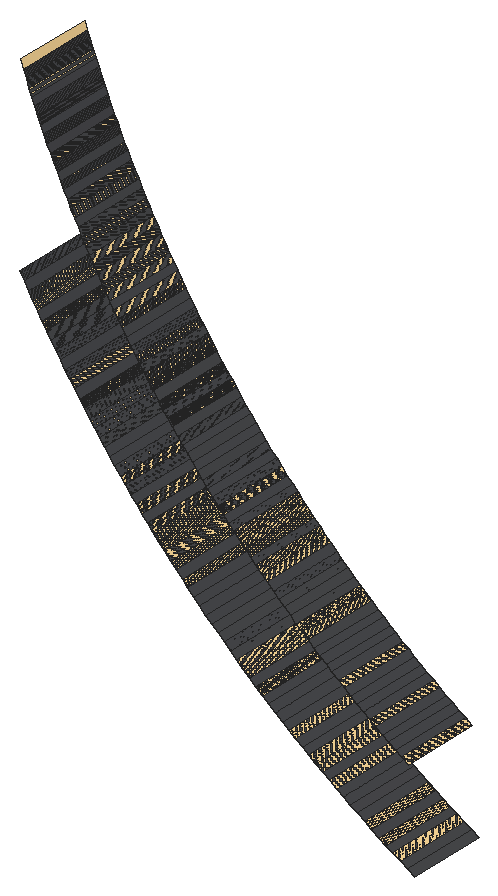
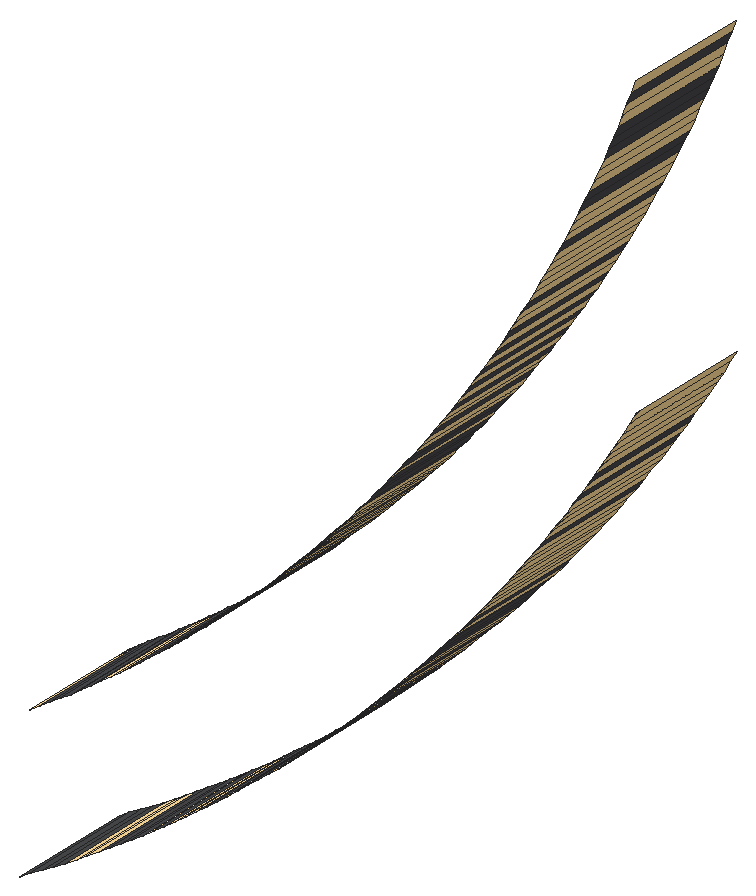
# SketchUp Ruby script. Lengths in inches.
U = 1.inch
M = Sketchup.active_model
def pt(a) = Geom::Point3d.new(a.map { |v| v * U })
def face(e, loops, mat)
  f = e.add_face(loops[0].map { |a| pt(a) })
  loops[1..].each { |l| e.add_face(l.map { |a| pt(a) }).erase! }
  f.material = f.back_material = mat if mat
  f
end
# faces: each face lists its corners as indices into pts; further lists are holes
def faces(e, pts, list, mat = nil) = list.each { |f| face(e, (f[0].is_a?(Array) ? f : [f]).map { |l| l.map { |i| pts[i] } }, mat) }
# xy, xz, yz: faces in a plane at the given z, y or x. An outline is a flat list of corners, or four numbers for a rectangle; further outlines are holes
def ring(l) = l.size == 4 ? [[l[0], l[1]], [l[2], l[1]], [l[2], l[3]], [l[0], l[3]]] : l.each_slice(2).to_a
def flat(e, list, mat, &to3) = list.each { |f| face(e, (f[0].is_a?(Array) ? f : [f]).map { |l| ring(l).map { |u, v| to3.(u, v) } }, mat) }
def xy(e, z, list, mat = nil) = flat(e, list, mat) { |x, y| [x, y, z] }
def xz(e, y, list, mat = nil) = flat(e, list, mat) { |x, z| [x, y, z] }
def yz(e, x, list, mat = nil) = flat(e, list, mat) { |y, z| [x, y, z] }
def lines(e, pts, list) = list.each { |a, b| e.add_line(pt(pts[a]), pt(pts[b])) }
# prism: a flat outline (further loops are holes) pulled along v
def prism(e, loops, v, mat = nil)
  f = face(e, loops, mat); d = Geom::Vector3d.new(v.map { |x| x * U })
  f.pushpull(f.normal.samedirection?(d) ? d.length : -d.length)
end
def box(e, o, s, mat = nil) = prism(e, [[o, [o[0] + s[0], o[1], o[2]], [o[0] + s[0], o[1] + s[1], o[2]], [o[0], o[1] + s[1], o[2]]]], [0, 0, s[2]], mat)
def at(x, y, z, deg = 0) = Geom::Transformation.translation(pt([x, y, z])) * Geom::Transformation.rotation(ORIGIN, Z_AXIS, deg.degrees)
def axes(o, x, y, z) = Geom::Transformation.new([*x, 0, *y, 0, *z, 0, *pt(o).to_a, 1])
def part(name) = M.definitions.add(name)
# library, detail: a bought-in or finely detailed component or shape, given as its bounding box
def library(name, o, s) = part(name).tap { |d| box(d.entities, o, s) }
def detail(e, o, s) = box(e.add_group.entities, o, s)
def put(e, d, t, mat = nil) = e.add_instance(d, t).tap { |i| i.material = mat if mat }
def group(e, t, mat = nil) = e.add_group.tap { |g| g.transformation = t; g.material = mat if mat }.entities
root = M.entities
M.materials.add("1432 AP 8245 TAR ROAD").color = [71, 72, 75]
M.materials.add("Outer Light").color = [251, 217, 152]
p = [[268.43,95.37,447.23],[268.56,95.37,447.15],[268.56,96.87,447.15],[268.43,96.87,447.23],[268.29,95.37,447.3125],[268.29,96.87,447.3125],
  [268.29,96.87,447.3125],[268.43,96.87,447.23],[268.43,95.37,447.23],[268.29,95.37,447.3125],[268.15,95.37,447.4],[268.15,96.87,447.4],
  [268.15,96.87,447.4],[268.15,95.37,447.4],[268.02,95.37,447.48],[268.02,96.87,447.48],[268.02,96.87,447.48],[268.02,95.37,447.48],
  [267.88,95.37,447.57],[267.88,96.87,447.57],[267.88,96.87,447.57],[267.88,95.37,447.57],[267.75,95.37,447.66],[267.75,96.87,447.66],
  [267.75,96.87,447.66],[267.75,95.37,447.66],[267.48,95.37,447.84],[267.61,95.37,447.75],[267.61,96.87,447.75],[267.48,96.87,447.84],
  [267.48,96.87,447.84],[267.61,96.87,447.75],[267.61,95.37,447.75],[267.48,95.37,447.84],[267.34,95.37,447.93],[267.34,96.87,447.93],
  [267.34,96.87,447.93],[267.34,95.37,447.93],[267.21,95.37,448.02],[267.21,96.87,448.02],[267.21,96.87,448.02],[267.21,95.37,448.02],
  [267.08,95.37,448.11],[267.08,96.87,448.11],[267.08,96.87,448.11],[267.08,95.37,448.11],[266.95,95.37,448.21],[266.95,96.87,448.21],
  [266.95,96.87,448.21],[266.95,95.37,448.21],[266.82,95.37,448.3],[266.82,96.87,448.3],[266.82,96.87,448.3],[266.82,95.37,448.3],
  [266.69,95.37,448.4],[266.69,96.87,448.4],[266.69,96.87,448.4],[266.69,95.37,448.4],[266.5625,95.37,448.5],[266.5625,96.87,448.5],
  [266.5625,96.87,448.5],[266.5625,95.37,448.5],[266.44,95.37,448.59],[266.44,96.87,448.59],[266.44,96.87,448.59],[266.44,95.37,448.59],
  [266.31,95.37,448.69],[266.31,96.87,448.69],[266.31,96.87,448.69],[266.31,95.37,448.69],[266.18,95.37,448.79],[266.18,96.87,448.79],
  [266.18,96.87,448.79],[266.18,95.37,448.79],[266.06,95.37,448.89],[266.06,96.87,448.89],[266.06,96.87,448.89],[266.06,95.37,448.89],
  [265.93,95.37,449],[265.93,96.87,449],[265.93,96.87,449],[265.93,95.37,449],[265.81,95.37,449.1],[265.81,96.87,449.1],
  [265.81,96.87,449.1],[265.81,95.37,449.1],[268.44,96.87,448.99],[268.32,96.87,449.08],[268.32,95.37,449.08],[268.44,95.37,448.99],
  [268.44,95.37,448.99],[268.32,95.37,449.08],[268.32,96.87,449.08],[268.44,96.87,448.99],[265.6875,95.37,449.2],[265.6875,96.87,449.2],
  [265.6875,96.87,449.2],[265.6875,95.37,449.2],[268.2,96.87,449.16],[268.2,95.37,449.16],[268.2,95.37,449.16],[268.2,96.87,449.16],
  [265.5625,95.37,449.31],[265.5625,96.87,449.31],[265.5625,96.87,449.31],[265.5625,95.37,449.31],[268.07,96.87,449.25],[267.95,96.87,449.33],
  [267.95,95.37,449.33],[268.07,95.37,449.25],[268.07,95.37,449.25],[267.95,95.37,449.33],[267.95,96.87,449.33],[268.07,96.87,449.25],
  [265.44,95.37,449.41],[265.44,96.87,449.41],[265.44,96.87,449.41],[265.44,95.37,449.41],[267.83,96.87,449.42],[267.83,95.37,449.42],
  [267.83,95.37,449.42],[267.83,96.87,449.42],[265.32,95.37,449.52],[265.32,96.87,449.52],[265.32,96.87,449.52],[265.32,95.37,449.52],
  [267.71,96.87,449.51],[267.71,95.37,449.51],[267.71,95.37,449.51],[267.71,96.87,449.51],[265.2,95.37,449.63],[265.2,96.87,449.63],
  [265.2,96.87,449.63],[265.2,95.37,449.63],[267.59,96.87,449.6],[267.59,95.37,449.6],[267.59,95.37,449.6],[267.59,96.87,449.6],
  [265.08,95.37,449.74],[265.08,96.87,449.74],[265.08,96.87,449.74],[265.08,95.37,449.74],[267.47,96.87,449.6875],[267.47,95.37,449.6875],
  [267.47,95.37,449.6875],[267.47,96.87,449.6875],[264.97,95.37,449.85],[264.97,96.87,449.85],[264.97,96.87,449.85],[264.97,95.37,449.85],
  [267.35,96.87,449.78],[267.35,95.37,449.78],[267.35,95.37,449.78],[267.35,96.87,449.78],[264.85,95.37,449.96],[264.85,96.87,449.96],
  [264.85,96.87,449.96],[264.85,95.37,449.96],[267.24,96.87,449.87],[267.24,95.37,449.87],[267.24,95.37,449.87],[267.24,96.87,449.87],
  [267.12,96.87,449.96],[267.12,95.37,449.96],[267.12,95.37,449.96],[267.12,96.87,449.96],[264.73,95.37,450.07],[264.73,96.87,450.07],
  [264.73,96.87,450.07],[264.73,95.37,450.07],[267,96.87,450.06],[267,95.37,450.06],[267,95.37,450.06],[267,96.87,450.06],
  [264.62,95.37,450.18],[264.62,96.87,450.18],[264.62,96.87,450.18],[264.62,95.37,450.18],[266.89,96.87,450.15],[266.89,95.37,450.15],
  [266.89,95.37,450.15],[266.89,96.87,450.15],[264.5,95.37,450.3],[264.5,96.87,450.3],[264.5,96.87,450.3],[264.5,95.37,450.3],
  [266.77,96.87,450.25],[266.66,96.87,450.34],[266.66,95.37,450.34],[266.77,95.37,450.25],[266.77,95.37,450.25],[266.66,95.37,450.34],
  [266.66,96.87,450.34],[266.77,96.87,450.25],[264.39,95.37,450.41],[264.39,96.87,450.41],[264.39,96.87,450.41],[264.39,95.37,450.41],
  [266.55,96.87,450.44],[266.55,95.37,450.44],[266.55,95.37,450.44],[266.55,96.87,450.44],[264.28,95.37,450.53],[264.28,96.87,450.53],
  [264.28,96.87,450.53],[264.28,95.37,450.53],[266.44,96.87,450.54],[266.44,95.37,450.54],[266.44,95.37,450.54],[266.44,96.87,450.54],
  [264.17,95.37,450.64],[264.17,96.87,450.64],[264.17,96.87,450.64],[264.17,95.37,450.64],[266.32,96.87,450.64],[266.32,95.37,450.64],
  [266.32,95.37,450.64],[266.32,96.87,450.64],[264.06,95.37,450.76],[264.06,96.87,450.76],[264.06,96.87,450.76],[264.06,95.37,450.76],
  [266.21,96.87,450.74],[266.21,95.37,450.74],[266.21,95.37,450.74],[266.21,96.87,450.74],[266.1,96.87,450.84],[266.1,95.37,450.84],
  [266.1,95.37,450.84],[266.1,96.87,450.84],[263.95,95.37,450.875],[263.95,96.87,450.875],[263.95,96.87,450.875],[263.95,95.37,450.875],
  [265.99,96.87,450.94],[265.99,95.37,450.94],[265.99,95.37,450.94],[265.99,96.87,450.94],[263.84,95.37,451],[263.84,96.87,451],
  [263.84,96.87,451],[263.84,95.37,451],[265.89,96.87,451.04],[265.89,95.37,451.04],[265.89,95.37,451.04],[265.89,96.87,451.04],
  [263.73,95.37,451.11],[263.73,96.87,451.11],[263.73,96.87,451.11],[263.73,95.37,451.11],[265.78,96.87,451.15],[265.78,95.37,451.15],
  [265.78,95.37,451.15],[265.78,96.87,451.15],[263.62,95.37,451.24],[263.62,96.87,451.24],[263.62,96.87,451.24],[263.62,95.37,451.24],
  [265.67,96.87,451.25],[265.67,95.37,451.25],[265.67,95.37,451.25],[265.67,96.87,451.25],[263.52,95.37,451.36],[263.52,96.87,451.36],
  [263.52,96.87,451.36],[263.52,95.37,451.36],[265.56,96.87,451.36],[265.56,95.37,451.36],[265.56,95.37,451.36],[265.56,96.87,451.36],
  [263.41,95.37,451.48],[263.41,96.87,451.48],[263.41,96.87,451.48],[263.41,95.37,451.48],[265.46,96.87,451.46],[265.46,95.37,451.46],
  [265.46,95.37,451.46],[265.46,96.87,451.46],[263.31,95.37,451.6],[263.31,96.87,451.6],[263.31,96.87,451.6],[263.31,95.37,451.6],
  [265.36,96.87,451.57],[265.36,95.37,451.57],[265.36,95.37,451.57],[265.36,96.87,451.57],[263.2,95.37,451.72],[263.2,96.87,451.72],
  [263.2,96.87,451.72],[263.2,95.37,451.72],[265.25,96.87,451.68],[265.25,95.37,451.68],[265.25,95.37,451.68],[265.25,96.87,451.68],
  [263.1,95.37,451.85],[263.1,96.87,451.85],[263.1,96.87,451.85],[263.1,95.37,451.85],[265.15,96.87,451.79],[265.15,95.37,451.79],
  [265.15,95.37,451.79],[265.15,96.87,451.79],[263,95.37,451.97],[263,96.87,451.97],[263,96.87,451.97],[263,95.37,451.97],
  [265.05,96.87,451.89],[265.05,95.37,451.89],[265.05,95.37,451.89],[265.05,96.87,451.89],[264.95,96.87,452],[264.95,95.37,452],
  [264.95,95.37,452],[264.95,96.87,452],[262.9,95.37,452.1],[262.9,96.87,452.1],[262.9,96.87,452.1],[262.9,95.37,452.1],
  [264.85,96.87,452.12],[264.85,95.37,452.12],[264.85,95.37,452.12],[264.85,96.87,452.12],[262.8,95.37,452.23],[262.8,96.87,452.23],
  [262.8,96.87,452.23],[262.8,95.37,452.23],[264.75,96.87,452.23],[264.75,95.37,452.23],[264.75,95.37,452.23],[264.75,96.87,452.23],
  [262.7,95.37,452.36],[262.7,96.87,452.36],[262.7,96.87,452.36],[262.7,95.37,452.36],[264.65,96.87,452.34],[264.65,95.37,452.34],
  [264.65,95.37,452.34],[264.65,96.87,452.34],[264.55,96.87,452.45],[264.55,95.37,452.45],[264.55,95.37,452.45],[264.55,96.87,452.45],
  [262.61,95.37,452.48],[262.61,96.87,452.48],[262.61,96.87,452.48],[262.61,95.37,452.48],[262.51,95.37,452.61],[262.51,96.87,452.61],
  [262.51,96.87,452.61],[262.51,95.37,452.61],[264.46,96.87,452.57],[264.46,95.37,452.57],[264.46,95.37,452.57],[264.46,96.87,452.57],
  [262.42,95.37,452.74],[262.42,96.87,452.74],[262.42,96.87,452.74],[262.42,95.37,452.74],[264.36,96.87,452.68],[264.36,95.37,452.68],
  [264.36,95.37,452.68],[264.36,96.87,452.68],[262.32,95.37,452.875],[262.32,96.87,452.875],[262.32,96.87,452.875],[262.32,95.37,452.875],
  [264.27,96.87,452.8],[264.27,95.37,452.8],[264.27,95.37,452.8],[264.27,96.87,452.8],[264.17,96.87,452.91],[264.17,95.37,452.91],
  [264.17,95.37,452.91],[264.17,96.87,452.91],[262.23,95.37,453],[262.23,96.87,453],[262.23,96.87,453],[262.23,95.37,453],
  [264.08,96.87,453.03],[264.08,95.37,453.03],[264.08,95.37,453.03],[264.08,96.87,453.03],[262.14,95.37,453.14],[262.14,96.87,453.14],
  [262.14,96.87,453.14],[262.14,95.37,453.14],[263.99,96.87,453.15],[263.99,95.37,453.15],[263.99,95.37,453.15],[263.99,96.87,453.15],
  [262.04,95.37,453.27],[262.04,96.87,453.27],[262.04,96.87,453.27],[262.04,95.37,453.27],[263.9,96.87,453.27],[263.9,95.37,453.27],
  [263.9,95.37,453.27],[263.9,96.87,453.27],[261.95,95.37,453.4],[261.95,96.87,453.4],[261.95,96.87,453.4],[261.95,95.37,453.4],
  [263.81,96.87,453.38],[263.81,95.37,453.38],[263.81,95.37,453.38],[263.81,96.87,453.38],[261.87,95.37,453.54],[261.87,96.87,453.54],
  [261.87,96.87,453.54],[261.87,95.37,453.54],[263.72,96.87,453.5],[263.72,95.37,453.5],[263.72,95.37,453.5],[263.72,96.87,453.5],
  [261.78,95.37,453.67],[261.78,96.87,453.67],[261.78,96.87,453.67],[261.78,95.37,453.67],[263.63,96.87,453.625],[263.63,95.37,453.625],
  [263.63,95.37,453.625],[263.63,96.87,453.625],[263.54,96.87,453.75],[263.54,95.37,453.75],[263.54,95.37,453.75],[263.54,96.87,453.75],
  [261.69,95.37,453.81],[261.69,96.87,453.81],[261.69,96.87,453.81],[261.69,95.37,453.81],[263.46,96.87,453.87],[263.46,95.37,453.87],
  [263.46,95.37,453.87],[263.46,96.87,453.87],[261.61,95.37,453.94],[261.61,96.87,453.94],[261.61,96.87,453.94],[261.61,95.37,453.94],
  [261.52,95.37,454.08],[261.52,96.87,454.08],[261.52,96.87,454.08],[261.52,95.37,454.08],[263.37,96.87,453.99],[263.37,95.37,453.99],
  [263.37,95.37,453.99],[263.37,96.87,453.99],[263.29,96.87,454.11],[263.29,95.37,454.11],[263.29,95.37,454.11],[263.29,96.87,454.11],
  [261.4375,95.37,454.22],[261.4375,96.87,454.22],[261.4375,96.87,454.22],[261.4375,95.37,454.22],[263.2,96.87,454.24],[263.2,95.37,454.24],
  [263.2,95.37,454.24],[263.2,96.87,454.24],[261.35,95.37,454.36],[261.35,96.87,454.36],[261.35,96.87,454.36],[261.35,95.37,454.36],
  [263.12,96.87,454.36],[263.12,95.37,454.36],[263.12,95.37,454.36],[263.12,96.87,454.36],[261.27,95.37,454.5],[261.27,96.87,454.5],
  [261.27,96.87,454.5],[261.27,95.37,454.5],[263.04,96.87,454.49],[263.04,95.37,454.49],[263.04,95.37,454.49],[263.04,96.87,454.49],
  [261.19,95.37,454.64],[261.19,96.87,454.64],[261.19,96.87,454.64],[261.19,95.37,454.64],[262.96,96.87,454.61],[262.96,95.37,454.61],
  [262.96,95.37,454.61],[262.96,96.87,454.61],[261.11,95.37,454.78],[261.11,96.87,454.78],[261.11,96.87,454.78],[261.11,95.37,454.78],
  [262.88,96.87,454.74],[262.88,95.37,454.74],[262.88,95.37,454.74],[262.88,96.87,454.74],[262.8,96.87,454.86],[262.8,95.37,454.86],
  [262.8,95.37,454.86],[262.8,96.87,454.86],[262.72,96.87,454.99],[262.72,95.37,454.99],[262.72,95.37,454.99],[262.72,96.87,454.99],
  [262.65,96.87,455.12],[262.65,95.37,455.12],[262.65,95.37,455.12],[262.65,96.87,455.12],[262.57,96.87,455.25],[262.57,95.37,455.25],
  [262.57,95.37,455.25],[262.57,96.87,455.25],[262.5,96.87,455.38],[262.5,95.37,455.38],[262.5,95.37,455.38],[262.5,96.87,455.38],
  [262.42,96.87,455.51],[262.42,95.37,455.51],[262.42,95.37,455.51],[262.42,96.87,455.51],[262.35,96.87,455.64],[262.35,95.37,455.64],
  [262.35,95.37,455.64],[262.35,96.87,455.64],[262.28,96.87,455.77],[262.28,95.37,455.77],[262.28,95.37,455.77],[262.28,96.87,455.77],
  [262.21,96.87,455.9],[262.21,95.37,455.9],[262.21,95.37,455.9],[262.21,96.87,455.9],[262.14,96.87,456.03],[262.14,95.37,456.03],
  [262.14,95.37,456.03],[262.14,96.87,456.03],[262.07,96.87,456.17],[262.07,95.37,456.17],[262.07,95.37,456.17],[262.07,96.87,456.17],
  [262,96.87,456.3],[262,95.37,456.3],[262,95.37,456.3],[262,96.87,456.3],[261.9375,96.87,456.43],[261.9375,95.37,456.43],
  [261.9375,95.37,456.43],[261.9375,96.87,456.43],[261.87,96.87,456.57],[261.87,95.37,456.57],[261.87,95.37,456.57],[261.87,96.87,456.57],
  [261.81,96.87,456.7],[261.81,95.37,456.7],[261.81,95.37,456.7],[261.81,96.87,456.7],[261.75,96.87,456.84],[261.75,95.37,456.84],
  [261.75,95.37,456.84],[261.75,96.87,456.84],[261.68,96.87,456.97],[261.68,95.37,456.97],[261.68,95.37,456.97],[261.68,96.87,456.97],
  [261.62,96.87,457.11],[261.62,95.37,457.11],[261.62,95.37,457.11],[261.62,96.87,457.11],[261.5625,96.87,457.25],[261.5625,95.37,457.25],
  [261.5625,95.37,457.25],[261.5625,96.87,457.25],[261.5,96.87,457.38],[261.5,95.37,457.38],[261.5,95.37,457.38],[261.5,96.87,457.38],
  [261.45,96.87,457.52],[261.45,95.37,457.52],[261.45,95.37,457.52],[261.45,96.87,457.52],[261.39,96.87,457.66],[261.39,95.37,457.66],
  [261.39,95.37,457.66],[261.39,96.87,457.66],[261.33,96.87,457.8],[261.33,95.37,457.8],[261.33,95.37,457.8],[261.33,96.87,457.8],
  [261.28,96.87,457.9375],[261.28,95.37,457.9375],[261.28,95.37,457.9375],[261.28,96.87,457.9375],[261.23,96.87,458.08],[261.23,95.37,458.08],
  [261.23,95.37,458.08],[261.23,96.87,458.08],[261.17,96.87,458.22],[261.17,95.37,458.22],[261.17,95.37,458.22],[261.17,96.87,458.22],
  [261.125,96.87,458.36],[261.125,95.37,458.36]]
faces(root,p,[[0,1,2,3],[4,0,3,5],[10,4,5,11],[14,10,11,15],[18,14,15,19],[22,18,19,23],[26,27,28,29],[27,22,23,28],
  [34,26,29,35],[38,34,35,39],[42,38,39,43],[46,42,43,47],[50,46,47,51],[54,50,51,55],[58,54,55,59],[62,58,59,63],
  [66,62,63,67],[70,66,67,71],[74,70,71,75],[78,74,75,79],[82,78,79,83],[90,91,92,93],[94,82,83,95],[91,100,101,92],
  [102,94,95,103],[110,111,112,113],[100,110,113,101],[114,102,103,115],[111,120,121,112],[122,114,115,123],[120,128,129,121],[130,122,123,131],
  [128,136,137,129],[138,130,131,139],[136,144,145,137],[146,138,139,147],[144,152,153,145],[154,146,147,155],[152,160,161,153],[160,164,165,161],
  [166,154,155,167],[164,172,173,165],[174,166,167,175],[172,180,181,173],[182,174,175,183],[190,191,192,193],[180,190,193,181],[194,182,183,195],
  [191,200,201,192],[202,194,195,203],[200,208,209,201],[210,202,203,211],[208,216,217,209],[218,210,211,219],[216,224,225,217],[224,228,229,225],
  [230,218,219,231],[228,236,237,229],[238,230,231,239],[236,244,245,237],[246,238,239,247],[244,252,253,245],[254,246,247,255],[252,260,261,253],
  [262,254,255,263],[260,268,269,261],[270,262,263,271],[268,276,277,269],[278,270,271,279],[276,284,285,277],[286,278,279,287],[284,292,293,285],
  [294,286,287,295],[292,300,301,293],[302,294,295,303],[300,308,309,301],[308,312,313,309],[314,302,303,315],[312,320,321,313],[322,314,315,323],
  [320,328,329,321],[330,322,323,331],[328,336,337,329],[336,340,341,337],[342,330,331,343],[346,342,343,347],[340,352,353,341],[354,346,347,355],
  [352,360,361,353],[362,354,355,363],[360,368,369,361],[368,372,373,369],[374,362,363,375],[372,380,381,373],[382,374,375,383],[380,388,389,381],
  [390,382,383,391],[388,396,397,389],[398,390,391,399],[396,404,405,397],[406,398,399,407],[404,412,413,405],[414,406,407,415],[412,420,421,413],
  [420,424,425,421],[426,414,415,427],[424,432,433,425],[434,426,427,435],[438,434,435,439],[432,444,445,433],[444,448,449,445],[450,438,439,451],
  [448,456,457,449],[458,450,451,459],[456,464,465,457],[466,458,459,467],[464,472,473,465],[474,466,467,475],[472,480,481,473],[482,474,475,483],
  [480,488,489,481],[488,492,493,489],[492,496,497,493],[496,500,501,497],[500,504,505,501],[504,508,509,505],[508,512,513,509],[512,516,517,513],
  [516,520,521,517],[520,524,525,521],[524,528,529,525],[528,532,533,529],[532,536,537,533],[536,540,541,537],[540,544,545,541],[544,548,549,545],
  [548,552,553,549],[552,556,557,553],[556,560,561,557],[560,564,565,561],[564,568,569,565],[568,572,573,569],[572,576,577,573],[576,580,581,577],
  [580,584,585,581],[584,588,589,585],[588,592,593,589]],"1432 AP 8245 TAR ROAD")
faces(root,p,[[6,7,8,9],[12,6,9,13],[16,12,13,17],[20,16,17,21],[24,20,21,25],[30,31,32,33],[31,24,25,32],[36,30,33,37],
  [40,36,37,41],[44,40,41,45],[48,44,45,49],[52,48,49,53],[56,52,53,57],[60,56,57,61],[64,60,61,65],[68,64,65,69],
  [72,68,69,73],[76,72,73,77],[80,76,77,81],[84,80,81,85],[86,87,88,89],[96,84,85,97],[87,98,99,88],[104,96,97,105],
  [106,107,108,109],[98,106,109,99],[116,104,105,117],[107,118,119,108],[124,116,117,125],[118,126,127,119],[132,124,125,133],[126,134,135,127],
  [140,132,133,141],[134,142,143,135],[148,140,141,149],[142,150,151,143],[156,148,149,157],[150,158,159,151],[158,162,163,159],[168,156,157,169],
  [162,170,171,163],[176,168,169,177],[170,178,179,171],[184,176,177,185],[186,187,188,189],[178,186,189,179],[196,184,185,197],[187,198,199,188],
  [204,196,197,205],[198,206,207,199],[212,204,205,213],[206,214,215,207],[220,212,213,221],[214,222,223,215],[222,226,227,223],[232,220,221,233],
  [226,234,235,227],[240,232,233,241],[234,242,243,235],[248,240,241,249],[242,250,251,243],[256,248,249,257],[250,258,259,251],[264,256,257,265],
  [258,266,267,259],[272,264,265,273],[266,274,275,267],[280,272,273,281],[274,282,283,275],[288,280,281,289],[282,290,291,283],[296,288,289,297],
  [290,298,299,291],[304,296,297,305],[298,306,307,299],[306,310,311,307],[316,304,305,317],[310,318,319,311],[324,316,317,325],[318,326,327,319],
  [332,324,325,333],[326,334,335,327],[334,338,339,335],[344,332,333,345],[348,344,345,349],[338,350,351,339],[356,348,349,357],[350,358,359,351],
  [364,356,357,365],[358,366,367,359],[366,370,371,367],[376,364,365,377],[370,378,379,371],[384,376,377,385],[378,386,387,379],[392,384,385,393],
  [386,394,395,387],[400,392,393,401],[394,402,403,395],[408,400,401,409],[402,410,411,403],[416,408,409,417],[410,418,419,411],[418,422,423,419],
  [428,416,417,429],[422,430,431,423],[436,428,429,437],[440,436,437,441],[430,442,443,431],[442,446,447,443],[452,440,441,453],[446,454,455,447],
  [460,452,453,461],[454,462,463,455],[468,460,461,469],[462,470,471,463],[476,468,469,477],[470,478,479,471],[484,476,477,485],[478,486,487,479],
  [486,490,491,487],[490,494,495,491],[494,498,499,495],[498,502,503,499],[502,506,507,503],[506,510,511,507],[510,514,515,511],[514,518,519,515],
  [518,522,523,519],[522,526,527,523],[526,530,531,527],[530,534,535,531],[534,538,539,535],[538,542,543,539],[542,546,547,543],[546,550,551,547],
  [550,554,555,551],[554,558,559,555],[558,562,563,559],[562,566,567,563],[566,570,571,567],[570,574,575,571],[574,578,579,575],[578,582,583,579],
  [582,586,587,583],[586,590,591,587],[590,594,595,591]],"Outer Light")
